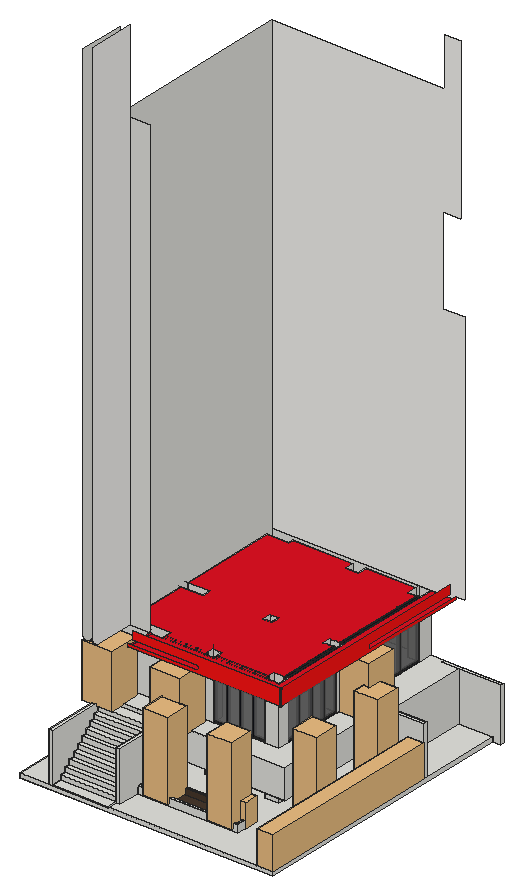
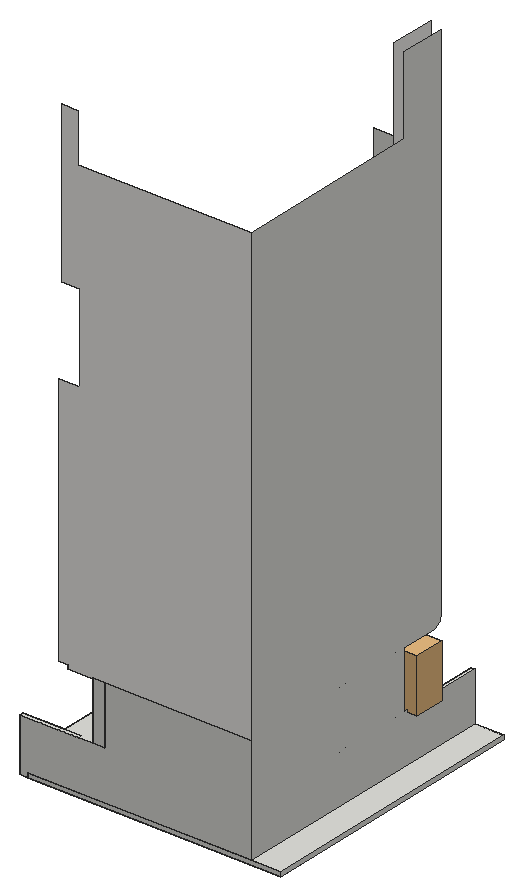
# SketchUp Ruby script. Lengths in inches.
U = 1.inch
M = Sketchup.active_model
def pt(a) = Geom::Point3d.new(a.map { |v| v * U })
def face(e, loops, mat)
  f = e.add_face(loops[0].map { |a| pt(a) })
  loops[1..].each { |l| e.add_face(l.map { |a| pt(a) }).erase! }
  f.material = f.back_material = mat if mat
  f
end
# faces: each face lists its corners as indices into pts; further lists are holes
def faces(e, pts, list, mat = nil) = list.each { |f| face(e, (f[0].is_a?(Array) ? f : [f]).map { |l| l.map { |i| pts[i] } }, mat) }
# xy, xz, yz: faces in a plane at the given z, y or x. An outline is a flat list of corners, or four numbers for a rectangle; further outlines are holes
def ring(l) = l.size == 4 ? [[l[0], l[1]], [l[2], l[1]], [l[2], l[3]], [l[0], l[3]]] : l.each_slice(2).to_a
def flat(e, list, mat, &to3) = list.each { |f| face(e, (f[0].is_a?(Array) ? f : [f]).map { |l| ring(l).map { |u, v| to3.(u, v) } }, mat) }
def xy(e, z, list, mat = nil) = flat(e, list, mat) { |x, y| [x, y, z] }
def xz(e, y, list, mat = nil) = flat(e, list, mat) { |x, z| [x, y, z] }
def yz(e, x, list, mat = nil) = flat(e, list, mat) { |y, z| [x, y, z] }
def lines(e, pts, list) = list.each { |a, b| e.add_line(pt(pts[a]), pt(pts[b])) }
# prism: a flat outline (further loops are holes) pulled along v
def prism(e, loops, v, mat = nil)
  f = face(e, loops, mat); d = Geom::Vector3d.new(v.map { |x| x * U })
  f.pushpull(f.normal.samedirection?(d) ? d.length : -d.length)
end
def box(e, o, s, mat = nil) = prism(e, [[o, [o[0] + s[0], o[1], o[2]], [o[0] + s[0], o[1] + s[1], o[2]], [o[0], o[1] + s[1], o[2]]]], [0, 0, s[2]], mat)
def at(x, y, z, deg = 0) = Geom::Transformation.translation(pt([x, y, z])) * Geom::Transformation.rotation(ORIGIN, Z_AXIS, deg.degrees)
def axes(o, x, y, z) = Geom::Transformation.new([*x, 0, *y, 0, *z, 0, *pt(o).to_a, 1])
def part(name) = M.definitions.add(name)
# library, detail: a bought-in or finely detailed component or shape, given as its bounding box
def library(name, o, s) = part(name).tap { |d| box(d.entities, o, s) }
def detail(e, o, s) = box(e.add_group.entities, o, s)
def put(e, d, t, mat = nil) = e.add_instance(d, t).tap { |i| i.material = mat if mat }
def group(e, t, mat = nil) = e.add_group.tap { |g| g.transformation = t; g.material = mat if mat }.entities
root = M.entities
M.materials.add("Generic").color = [242, 241, 238]
M.materials.add("Heather_Band").color = [255, 20, 20]
M.materials.add("Lisanne_Bandana").color = [222, 18, 34]
M.materials.add("Soil A01 200cm").color = [71, 56, 44]
M.materials.add("{045efeae-c101-a24d-bd9b-6f5600100adb}").color = [102, 102, 102]
M.materials["{045efeae-c101-a24d-bd9b-6f5600100adb}"].alpha = 0.7
M.materials.add("{16756a1b-d383-d94f-ad82-104813d2624f}").color = [19, 21, 27]
c1 = library("Vaso decorativo com seixos\#1",[6.14,-4.72,0],[9.45,4.72,3.26])
c2 = library("Artificial Plant-025",[-16.27,-15.82,25.53],[31.86,30.79,20.59])
c3 = library("Group4\#2",[-14.05,-12.91,-0.09],[26.62,27.13,73.11])
c4 = library("Plant\#1",[-27.84,-31.84,-1.26],[68.28,70.82,154.38])
c5 = part("Furniture_0DcpanrIvuI8n_9Ae92L5A")
g1 = group(c5.entities,at(0,0,0))
box(g1,[-19.29,-0.2,0.39],[38.58,0.4,83.86],"{045efeae-c101-a24d-bd9b-6f5600100adb}")
g2 = group(c5.entities,at(0,0,0))
box(g2,[-19.68,-0.59,63.39],[39.36,1.18,0.39],"{16756a1b-d383-d94f-ad82-104813d2624f}")
box(g2,[-19.68,-0.59,42.52],[39.36,1.18,0.39],"{16756a1b-d383-d94f-ad82-104813d2624f}")
box(g2,[-19.68,-0.59,21.26],[39.36,1.18,0.39],"{16756a1b-d383-d94f-ad82-104813d2624f}")
xy(g2,0,[[-19.68,-0.59,19.68,0.59]],"{16756a1b-d383-d94f-ad82-104813d2624f}")
xy(g2,0.39,[[-19.68,-0.59,-19.29,0.59],[-19.68,-0.59,19.68,0.59],[19.29,-0.59,19.68,0.59]],"{16756a1b-d383-d94f-ad82-104813d2624f}")
xy(g2,84.25,[[-19.68,-0.59,19.68,0.59]],"{16756a1b-d383-d94f-ad82-104813d2624f}")
xy(g2,84.65,[[-19.68,-0.59,-19.29,0.59],[-19.68,-0.59,19.68,0.59],[19.29,-0.59,19.68,0.59]],"{16756a1b-d383-d94f-ad82-104813d2624f}")
xz(g2,-0.59,[[-19.68,0,19.68,0.39],[-19.68,0.39,-19.29,84.65],[19.29,0.39,19.68,84.65],[-19.68,84.25,19.68,84.65]],"{16756a1b-d383-d94f-ad82-104813d2624f}")
xz(g2,0.59,[[-19.68,0,19.68,0.39],[-19.68,0.39,-19.29,84.65],[19.29,0.39,19.68,84.65],[-19.68,84.25,19.68,84.65]],"{16756a1b-d383-d94f-ad82-104813d2624f}")
yz(g2,-19.68,[[-0.59,0,0.59,0.39],[-0.59,0.39,0.59,84.65],[-0.59,84.25,0.59,84.65]],"{16756a1b-d383-d94f-ad82-104813d2624f}")
yz(g2,-19.29,[[-0.59,0.39,0.59,84.65]],"{16756a1b-d383-d94f-ad82-104813d2624f}")
yz(g2,19.29,[[-0.59,0.39,0.59,84.65]],"{16756a1b-d383-d94f-ad82-104813d2624f}")
yz(g2,19.68,[[-0.59,0,0.59,0.39],[-0.59,0.39,0.59,84.65],[-0.59,84.25,0.59,84.65]],"{16756a1b-d383-d94f-ad82-104813d2624f}")
c6 = part("Glass+Window")
put(c6.entities,c5,at(0,0,-42.32))
xy(root,-0.04,[[572.97,624.46,591.69,632.34]])
xy(root,0,[[0,0,572.97,632.34]])
xy(root,9.06,[[73.38,0,200.04,23.86]])
xy(root,9.63,[[0,0,65.42,632.34],[65.42,0,73.38,632.34],[[73.38,0,572.97,0,572.97,428.91,537.05,428.91,537.05,171.7,490.98,171.7,490.98,437.32,427.22,437.32,427.22,624.46,73.38,624.46],[200.04,21.81,200.04,122.47,438.39,122.47,438.39,70.9,209.88,70.9,209.88,21.81],[395.59,200.9,427.22,225.25],[395.59,366.03,427.22,385.17],[258.28,200.9,278.54,225.25]],[200.04,21.81,209.88,107.3],[209.88,70.9,438.39,122.47],
  [490.98,171.7,537.05,171.7,537.05,428.91,572.97,428.91,572.97,437.32,490.98,437.32],[258.28,200.9,278.54,225.25],[395.59,200.9,427.22,225.25],[395.59,366.03,427.22,385.17],[497.18,437.32,572.97,624.46],
  [73.38,624.46,572.97,632.34]])
xy(root,10.83,[[73.38,0,200.04,23.625]])
xy(root,13.19,[[215.62,76.64,432.66,116.73]],"Soil A01 200cm")
xy(root,17.94,[[499.14,179.86,528.9,420.75]],"Soil A01 200cm")
xy(root,21.22,[[73.38,23.625,200.04,35.4375]])
xy(root,25.69,[[[209.88,70.9,438.39,122.47],[215.62,76.64,432.66,116.73]],[200.04,122.47,209.88,139.96],[[490.98,171.7,537.05,428.91],[499.14,179.86,528.9,420.75]]])
xy(root,31.61,[[73.38,35.4375,200.04,47.25]])
xy(root,42,[[73.38,47.25,200.04,59.0625]])
xy(root,51.89,[[479.31,428.91,490.98,437.32]])
xy(root,52.39,[[73.38,59.0625,200.04,70.875]])
xy(root,54.09,[[200.04,139.96,209.88,153.5625],[73.38,153.5625,200.04,200.9],[200.04,153.5625,209.88,200.9],[209.88,153.5625,209.88,200.9,427.22,200.9,427.22,437.32,479.31,437.32,479.31,153.5625]])
xy(root,62.78,[[73.38,70.875,200.04,82.6875]])
xy(root,69.75,[[73.38,200.9,73.38,624.46,427.22,624.46,427.22,385.17,395.59,385.17,395.59,366.03,427.22,366.03,427.22,225.25,395.59,225.25,395.59,200.9,278.54,200.9,278.54,225.25,258.28,225.25,258.28,200.9],[258.28,200.9,278.54,225.25]])
xy(root,73.17,[[73.38,82.6875,200.04,94.5]])
xy(root,83.56,[[73.38,94.5,200.04,106.3125]])
xy(root,93.95,[[73.38,106.3125,200.04,118.125]])
xy(root,104.34,[[73.38,118.125,200.04,129.9375]])
xy(root,112.96,[[73.38,141.98,200.04,153.5625]])
xy(root,114.73,[[73.38,129.9375,200.04,153.5625]])
xy(root,121.46,[[200.04,21.81,209.88,153.5625],[[65.42,153.5625,479.31,153.5625,479.31,428.91,457.86,428.91,457.86,437.32,497.18,437.32,497.18,624.46,457.86,624.46,457.86,632.34,427.22,632.34,427.22,601.16,399.86,601.16,399.86,624.18,286.77,623.03,286.77,601.16,258.28,601.16,258.28,622.73,122.07,621.34,122.07,610.34,72.25,610.34,72.25,385.17,122.07,385.17,122.07,366.03,72.25,366.03,72.25,225.25,161.48,225.25,161.48,200.9,65.42,200.9],[395.59,200.9,427.22,225.25],[395.59,366.03,427.22,385.17],[258.28,200.9,278.54,225.25],[258.28,366.03,278.54,385.17]],[133.86,200.9,161.48,225.25],[258.28,200.9,278.54,225.25],[395.59,200.9,427.22,225.25],
  [72.25,366.03,122.07,385.17],[457.86,428.91,572.97,437.32],[258.28,601.16,286.77,601.16,286.77,623.03,258.28,622.73],[399.86,601.16,399.86,624.18,427.22,624.46,427.22,601.16],[399.86,624.18,399.86,632.34,427.22,632.34,427.22,624.46],
  [457.86,624.46,591.69,632.34]])
xy(root,252.9,[[65.42,117.34,87.56,200.9]])
xy(root,252.9,[[[137.05,137.375,137.05,200.9,161.48,200.9,161.48,225.25,72.25,225.25,72.25,366.03,122.07,366.03,122.07,385.17,72.25,385.17,72.25,610.34,122.07,610.34,122.07,621.34,258.28,622.73,258.28,601.16,286.77,601.16,286.77,623.03,399.86,624.18,399.86,601.16,427.22,601.16,427.22,632.34,482.71,632.34,482.71,140.59,482.6875,140.17,482.6,139.75,482.47,139.36,482.28,138.98,482.05,138.63,481.77,138.32,481.46,138.04,481.11,137.81,480.73,137.62,480.33,137.49,479.92,137.4,479.5,137.375],[395.59,200.9,427.22,225.25],[395.59,366.03,427.22,385.17],[258.28,200.9,278.54,225.25],[258.28,366.03,278.54,385.17]]],"Lisanne_Bandana")
xz(root,0,[[0,0,572.97,0,572.97,9.63,200.04,9.63,200.04,9.06,73.38,9.06,73.38,9.63,0,9.63],[73.38,9.06,200.04,9.63],[65.42,9.63,73.38,121.45],[73.38,9.63,200.04,10.83]])
xz(root,21.81,[[200.04,9.63,209.88,121.46]])
xz(root,23.625,[[73.38,10.83,200.04,21.22]])
xz(root,35.4375,[[73.38,21.22,200.04,31.61]])
xz(root,47.25,[[73.38,31.61,200.04,42]])
xz(root,59.0625,[[73.38,42,200.04,52.39]])
xz(root,70.875,[[73.38,52.39,200.04,62.78]])
xz(root,70.9,[[209.88,9.63,438.39,25.69]])
xz(root,76.64,[[215.62,13.19,432.66,25.69]],"Soil A01 200cm")
xz(root,82.6875,[[73.38,62.78,200.04,73.17]])
xz(root,94.5,[[73.38,73.17,200.04,83.56]])
xz(root,106.3125,[[73.38,83.56,200.04,93.95]])
xz(root,116.73,[[215.62,13.19,432.66,25.69]],"Soil A01 200cm")
xz(root,118.125,[[73.38,93.95,200.04,104.34]])
xz(root,122.47,[[200.04,9.63,209.88,25.69],[209.88,9.63,438.39,25.69]])
xz(root,129.9375,[[73.38,104.34,200.04,114.73]])
xz(root,137.375,[[137.05,252.9,479.5,252.9,479.5,289.68,145.77,289.68,145.77,270.88,291.875,270.88,292.42,270.85,292.96,270.77,293.49,270.625,294,270.43,294.49,270.18,294.95,269.88,295.37,269.54,295.76,269.15,296.1,268.73,296.4,268.27,296.65,267.78,296.84,267.27,296.99,266.74,297.07,266.2,297.1,265.66,297.07,265.11,296.99,264.57,296.84,264.04,296.65,263.53,296.4,263.05,296.1,262.59,295.76,262.16,295.37,261.78,294.95,261.43,294.49,261.13,294,260.89,293.49,260.6875,292.96,260.55,292.42,260.46,291.875,260.43,136.89,260.43,135.9375,260.11,135.1,259.56,134.44,258.81,133.99,257.91,133.86,257.23,133.86,255.93,134.18,254.98,134.74,254.14,135.49,253.48,136.39,253.03]],"Heather_Band")
xz(root,139.96,[[200.04,25.69,209.88,54.09]])
xz(root,153.5625,[[73.38,54.09,200.04,112.96],[200.04,54.09,209.88,121.46],[209.88,54.09,479.31,121.46],[73.38,112.96,200.04,114.73],[73.38,114.73,200.04,121.46]])
xz(root,171.7,[[490.98,9.63,537.05,25.69]])
xz(root,179.86,[[499.14,17.94,528.9,25.69]],"Soil A01 200cm")
xz(root,200.9,[[258.28,9.63,278.54,54.09],[395.59,9.63,427.22,54.09],[73.38,54.09,200.04,69.75],[200.04,54.09,209.88,69.75],[209.88,54.09,258.28,69.75],
  [258.28,54.09,278.54,69.75],[278.54,54.09,395.59,69.75],[65.42,121.46,161.48,121.46,161.48,252.9,137.05,252.9,136.39,253.03,135.49,253.48,134.74,254.14,134.18,254.98,133.86,255.93,133.86,255.95,133.86,252.9,65.42,252.9],[258.28,121.46,278.54,252.9],[395.59,121.46,427.22,252.9],
  [87.56,252.9,133.86,252.9,133.86,257.23,133.99,257.91,134.44,258.81,135.1,259.56,135.9375,260.11,136.89,260.43,133.86,260.43,133.86,1286.04,87.56,1286.04]])
xz(root,225.25,[[258.28,9.63,278.54,69.75],[395.59,9.63,427.22,69.75],[258.28,69.75,278.54,121.46],[72.25,121.46,161.48,252.9],[258.28,121.46,278.54,252.9],
  [395.59,121.46,427.22,252.9]])
xz(root,366.03,[[395.59,9.63,427.22,69.75],[395.59,69.75,427.22,121.46],[72.25,121.46,122.07,252.9],[258.28,121.46,278.54,252.9],[395.59,121.46,427.22,252.9]])
xz(root,385.17,[[395.59,9.63,427.22,69.75],[395.59,69.75,427.22,121.46],[72.25,121.46,122.07,252.9],[258.28,121.46,278.54,252.9],[395.59,121.46,427.22,252.9]])
xz(root,420.75,[[499.14,17.94,528.9,25.69]],"Soil A01 200cm")
xz(root,428.91,[[537.05,9.63,572.97,9.63,572.97,121.46,479.31,121.46,479.31,51.89,490.98,51.89,490.98,25.69,537.05,25.69]])
xz(root,437.32,[[427.22,9.63,455.29,54.09],[455.29,9.63,490.98,9.63,490.98,51.89,479.31,51.89,479.31,54.09,455.29,54.09],[490.98,9.63,490.98,51.89,479.31,51.89,479.31,54.09,497.18,54.09,497.18,9.63],[497.18,9.63,572.97,121.46]])
xz(root,601.16,[[258.28,121.46,286.77,252.9],[399.86,121.46,427.22,252.9]])
xz(root,610.34,[[72.25,121.46,122.07,252.9]])
xz(root,624.46,[[572.97,-0.04,591.69,-0.04,591.69,121.46,497.18,121.46,497.18,9.63,572.97,9.63],[73.38,9.63,427.22,69.75]])
xz(root,632.34,[[572.97,-0.04,572.97,9.63,65.42,9.63,65.42,252.9,399.86,252.9,399.86,121.46,591.69,121.46,591.69,-0.04],[0,0,572.97,9.63],[399.86,121.46,427.22,252.9]])
xz(root,632.34,[[65.42,252.9,65.42,1286.04,459.56,1286.04,459.56,1395.5,495.7,1395.5,495.7,1033.75,454.94,1033.75,454.94,835.52,503.14,835.52,503.14,260.43,482.71,260.43,482.71,252.9]],"Generic")
yz(root,0,[[0,0,632.34,9.63]])
yz(root,65.42,[[0,9.63,0,121.45,153.5625,121.46,200.9,121.46,200.9,252.9,117.34,252.9,114.59,253.08,111.88,253.62,109.26,254.51,106.79,255.73,104.49,257.26,102.42,259.08,100.6,261.16,99.07,263.45,97.85,265.93,96.96,268.54,96.42,271.25,96.24,274,96.24,1463.08,200.9,1463.08,200.9,1286.04,632.34,1286.04,632.34,9.63]])
yz(root,72.25,[[225.25,121.46,366.03,252.9],[385.17,121.46,610.34,252.9]])
yz(root,73.38,[[0,9.06,0,9.63,24.51,9.63,23.86,9.06],[0,9.63,0,10.83,23.625,10.83,23.625,21.22,35.4375,21.22,35.4375,31.61,47.25,31.61,47.25,42,59.0625,42,59.0625,52.39,70.875,52.39,70.875,62.78,82.6875,62.78,82.6875,73.17,94.5,73.17,94.5,83.56,106.3125,83.56,106.3125,93.95,118.125,93.95,118.125,104.34,129.9375,104.34,129.9375,114.73,153.5625,114.73,153.5625,112.96,141.98,112.96,24.51,9.63],[24.51,9.63,624.46,9.63,624.46,69.75,200.9,69.75,200.9,54.09,153.5625,54.09,153.5625,112.96,141.98,112.96],[0,10.83,23.625,10.83,23.625,21.22,35.4375,21.22,35.4375,31.61,47.25,31.61,47.25,42,59.0625,42,59.0625,52.39,70.875,52.39,70.875,62.78,82.6875,62.78,82.6875,73.17,94.5,73.17,94.5,83.56,106.3125,83.56,106.3125,93.95,118.125,93.95,118.125,104.34,129.9375,104.34,129.9375,114.73,153.5625,114.73,153.5625,121.46,0,121.45]])
yz(root,87.56,[[117.34,252.9,200.9,252.9,200.9,1474.125,96.24,1474.125,96.24,274,96.42,271.25,96.96,268.54,97.85,265.93,99.07,263.45,100.6,261.16,102.42,259.08,104.49,257.26,106.79,255.73,109.26,254.51,111.88,253.62,114.59,253.08]],"Generic")
yz(root,122.07,[[366.03,121.46,385.17,252.9],[610.34,121.46,621.34,252.9]])
yz(root,161.48,[[200.9,121.46,225.25,252.9]])
yz(root,200.04,[[0,9.06,23.86,9.06,24.51,9.63,21.81,9.63,21.81,10.83,0,10.83],[21.81,9.63,21.81,10.83,23.625,10.83,23.625,21.22,35.4375,21.22,35.4375,31.61,47.25,31.61,47.25,42,59.0625,42,59.0625,52.39,70.875,52.39,70.875,62.78,82.6875,62.78,82.6875,73.17,94.5,73.17,94.5,83.56,106.3125,83.56,106.3125,93.95,118.125,93.95,118.125,104.34,129.9375,104.34,129.9375,114.73,153.5625,114.73,153.5625,112.96,141.98,112.96,24.51,9.63],[24.51,9.63,141.98,112.96,153.5625,112.96,153.5625,54.09,139.96,54.09,139.96,25.69,122.47,25.69,122.47,9.63],[21.81,10.83,21.81,121.46,153.5625,121.46,153.5625,114.73,129.9375,114.73,129.9375,104.34,118.125,104.34,118.125,93.95,106.3125,93.95,106.3125,83.56,94.5,83.56,94.5,73.17,82.6875,73.17,82.6875,62.78,70.875,62.78,70.875,52.39,59.0625,52.39,59.0625,42,47.25,42,47.25,31.61,35.4375,31.61,35.4375,21.22,23.625,21.22,23.625,10.83]])
yz(root,209.88,[[21.81,9.63,70.9,9.63,70.9,25.69,139.96,25.69,139.96,54.09,153.5625,54.09,153.5625,121.46,21.81,121.46],[70.9,9.63,122.47,25.69]])
yz(root,215.62,[[76.64,13.19,116.73,25.69]],"Soil A01 200cm")
yz(root,258.28,[[200.9,9.63,225.25,69.75],[200.9,121.46,225.25,252.9],[366.03,121.46,385.17,252.9],[601.16,121.46,622.73,252.9]])
yz(root,278.54,[[200.9,9.63,225.25,69.75],[200.9,121.46,225.25,252.9],[366.03,121.46,385.17,252.9]])
yz(root,286.77,[[601.16,121.46,623.03,252.9]])
yz(root,395.59,[[200.9,9.63,225.25,69.75],[366.03,9.63,385.17,69.75],[200.9,69.75,225.25,121.46],[366.03,69.75,385.17,121.46],[200.9,121.46,225.25,252.9],
  [366.03,121.46,385.17,252.9]])
yz(root,399.86,[[601.16,121.46,624.18,252.9],[624.18,121.46,632.34,252.9]])
yz(root,427.22,[[200.9,9.63,225.25,54.09],[366.03,9.63,385.17,54.09],[437.32,9.63,624.46,69.75],[225.25,54.09,366.03,69.75],[366.03,54.09,385.17,121.46],
  [385.17,54.09,428.91,69.75],[428.91,54.09,437.32,69.75],[200.9,121.46,225.25,252.9],[366.03,121.46,385.17,252.9],[601.16,121.46,632.34,252.9]])
yz(root,432.66,[[76.64,13.19,116.73,25.69]])
yz(root,438.39,[[70.9,9.63,122.47,25.69]])
yz(root,479.31,[[428.91,51.89,437.32,54.09],[153.5625,54.09,428.91,121.46]])
yz(root,482.71,[[140.59,252.9,632.34,252.9,632.34,260.43,389.19,260.43,388.71,260.53,388.25,260.68,387.79,260.86,387.36,261.09,386.95,261.36,386.57,261.67,386.22,262.01,385.9,262.375,385.625,262.78,385.38,263.2,385.18,263.65,385.02,264.11,384.91,264.58,384.84,265.07,384.82,265.56,384.84,266.04,384.91,266.53,385.02,267,385.18,267.46,385.38,267.91,385.625,268.33,385.9,268.73,386.22,269.11,386.57,269.45,386.95,269.75,387.36,270.02,387.79,270.25,388.25,270.43,388.71,270.58,389.19,270.68,617.58,270.68,617.58,289.68,140.59,289.68]],"Heather_Band")
yz(root,490.98,[[171.7,9.63,171.7,25.69,428.91,25.69,428.91,51.89,437.32,51.89,437.32,9.63]])
yz(root,497.18,[[437.32,9.63,624.46,121.46]])
yz(root,499.14,[[179.86,17.94,420.75,25.69]],"Soil A01 200cm")
yz(root,528.9,[[179.86,17.94,420.75,25.69]],"Soil A01 200cm")
yz(root,537.05,[[171.7,9.63,428.91,25.69]])
yz(root,572.97,[[624.46,-0.04,632.34,0],[0,0,624.46,9.63],[624.46,0,632.34,9.63],[428.91,9.63,437.32,121.46]])
yz(root,591.69,[[624.46,-0.04,632.34,121.46]])
p = [[73.38,24.51,9.63],[73.38,141.98,112.96],[200.04,141.98,112.96],[200.04,24.51,9.63],[200.04,23.86,9.06],[73.38,23.86,9.06],
  [73.38,0,121.45],[73.38,153.5625,121.46],[65.42,153.5625,121.46],[65.42,0,121.45],[122.07,621.34,121.46],[258.28,622.73,121.46],
  [258.28,622.73,252.9],[122.07,621.34,252.9],[286.77,623.03,121.46],[399.86,624.18,121.46],[399.86,624.18,252.9],[286.77,623.03,252.9],
  [87.56,117.34,252.9],[87.56,114.59,253.08],[65.42,114.59,253.08],[65.42,117.34,252.9],[137.05,137.375,252.9],[136.39,137.375,253.03],
  [136.39,200.9,253.03],[137.05,200.9,252.9],[479.5,137.375,252.9],[479.92,137.4,252.9],[479.92,137.4,289.68],[479.5,137.375,289.68],
  [480.33,137.49,252.9],[480.33,137.49,289.68],[480.73,137.62,252.9],[480.73,137.62,289.68],[481.11,137.81,252.9],[481.11,137.81,289.68],
  [481.46,138.04,252.9],[481.46,138.04,289.68],[481.77,138.32,252.9],[481.77,138.32,289.68],[482.05,138.63,252.9],[482.05,138.63,289.68],
  [482.28,138.98,252.9],[482.28,138.98,289.68],[482.47,139.36,252.9],[482.47,139.36,289.68],[482.6,139.75,252.9],[482.6,139.75,289.68],
  [482.6875,140.17,252.9],[482.6875,140.17,289.68],[482.71,140.59,252.9],[482.71,140.59,289.68],[135.49,137.375,253.48],[135.49,200.9,253.48],
  [87.56,111.88,253.62],[65.42,111.88,253.62],[134.74,137.375,254.14],[134.74,200.9,254.14],[87.56,109.26,254.51],[65.42,109.26,254.51],
  [65.42,225.25,121.46],[72.25,225.25,121.46],[258.28,225.25,252.9],[258.28,225.25,261.99],[427.22,428.91,121.46],[427.22,428.91,69.75],
  [209.88,139.96,9.63],[209.88,139.96,6.84],[72.25,385.17,121.46],[65.42,385.17,121.46],[72.25,366.03,121.46],[65.42,366.03,121.46],
  [72.25,385.17,252.9],[65.42,385.17,252.9],[72.25,225.25,252.9],[65.42,225.25,252.9],[72.25,366.03,252.9],[65.42,366.03,252.9]]
faces(root,p,[[0,1,2,3,4,5],[6,7,8,9],[10,11,12,13],[14,15,16,17]])
faces(root,p,[[18,19,20,21],[19,54,55,20],[54,58,59,55]],"Generic")
faces(root,p,[[22,23,24,25],[26,27,28,29],[27,30,31,28],[30,32,33,31],[32,34,35,33],[34,36,37,35],[36,38,39,37],[38,40,41,39],
  [40,42,43,41],[42,44,45,43],[44,46,47,45],[46,48,49,47],[48,50,51,49],[23,52,53,24],[52,56,57,53]],"Lisanne_Bandana")
lines(root,p,[[60,61],[62,63],[64,65],[66,67],[68,69],[70,71],[72,73],[74,75],[76,77]])
put(root,c1,axes([537.05,-278.42,9.63],[0,45.36882,0],[-7.67077,0,0],[0,0,22.7292]))
put(root,c2,axes([422.81,107.49,-56.53],[1,0,0],[0,1,0],[0,0,2.5917]))
put(root,c3,axes([253.56,93.76,13.41],[2.1,0,0],[0,2.0184,0],[0,0,2.42]))
put(root,c3,axes([400.06,93.76,13.41],[2.1,0,0],[0,2.0184,0],[0,0,2.42]))
put(root,c3,axes([510.99,199.78,17.78],[0,2.1,0],[-2.0184,0,0],[0,0,2.42]))
put(root,c3,axes([510.99,374.9,17.78],[0,2.1,0],[-2.0184,0,0],[0,0,2.42]))
put(root,c4,axes([69.46,154.2,119.54],[1,0,0],[0,1,0],[0,0,0.79]))
put(root,c4,axes([223.77,154.2,119.54],[1,0,0],[0,1,0],[0,0,0.79]))
put(root,c4,axes([454.78,403.4,121.12],[1,0,0],[0,1,0],[0,0,0.79]))
put(root,c6,axes([209.88,206.22,186.98],[0,0,-3.34871],[0,-7,0],[1.14361,0,0]))
put(root,c6,axes([337.07,206.22,186.98],[0,0,-3.34871],[0,-7,0],[1.38289,0,0]))
put(root,c6,axes([423.08,493.17,187.375],[0,0,-3.34871],[7,0,0],[0,2.55169,0]))
put(root,c6,axes([423.08,295.64,187.375],[0,0,-3.34871],[7,0,0],[0,1.66315,0]))
